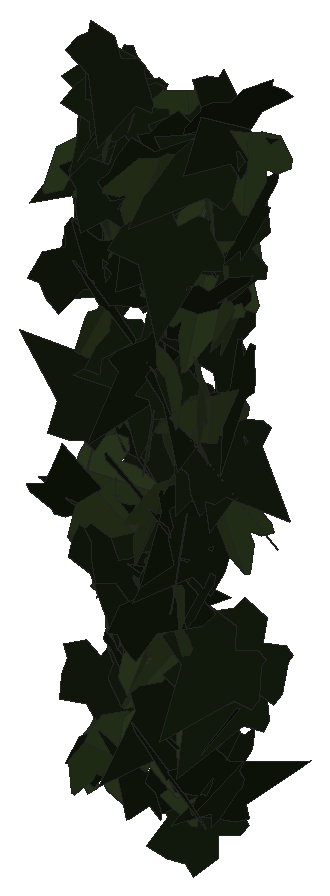
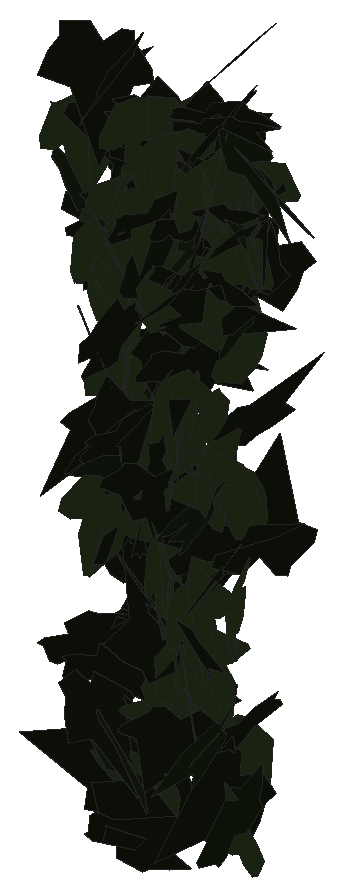
# SketchUp Ruby script. Lengths in inches.
U = 1.inch
M = Sketchup.active_model
def pt(a) = Geom::Point3d.new(a.map { |v| v * U })
def face(e, loops, mat)
  f = e.add_face(loops[0].map { |a| pt(a) })
  loops[1..].each { |l| e.add_face(l.map { |a| pt(a) }).erase! }
  f.material = f.back_material = mat if mat
  f
end
# faces: each face lists its corners as indices into pts; further lists are holes
def faces(e, pts, list, mat = nil) = list.each { |f| face(e, (f[0].is_a?(Array) ? f : [f]).map { |l| l.map { |i| pts[i] } }, mat) }
# xy, xz, yz: faces in a plane at the given z, y or x. An outline is a flat list of corners, or four numbers for a rectangle; further outlines are holes
def ring(l) = l.size == 4 ? [[l[0], l[1]], [l[2], l[1]], [l[2], l[3]], [l[0], l[3]]] : l.each_slice(2).to_a
def flat(e, list, mat, &to3) = list.each { |f| face(e, (f[0].is_a?(Array) ? f : [f]).map { |l| ring(l).map { |u, v| to3.(u, v) } }, mat) }
def xy(e, z, list, mat = nil) = flat(e, list, mat) { |x, y| [x, y, z] }
def xz(e, y, list, mat = nil) = flat(e, list, mat) { |x, z| [x, y, z] }
def yz(e, x, list, mat = nil) = flat(e, list, mat) { |y, z| [x, y, z] }
def lines(e, pts, list) = list.each { |a, b| e.add_line(pt(pts[a]), pt(pts[b])) }
# prism: a flat outline (further loops are holes) pulled along v
def prism(e, loops, v, mat = nil)
  f = face(e, loops, mat); d = Geom::Vector3d.new(v.map { |x| x * U })
  f.pushpull(f.normal.samedirection?(d) ? d.length : -d.length)
end
def box(e, o, s, mat = nil) = prism(e, [[o, [o[0] + s[0], o[1], o[2]], [o[0] + s[0], o[1] + s[1], o[2]], [o[0], o[1] + s[1], o[2]]]], [0, 0, s[2]], mat)
def at(x, y, z, deg = 0) = Geom::Transformation.translation(pt([x, y, z])) * Geom::Transformation.rotation(ORIGIN, Z_AXIS, deg.degrees)
def axes(o, x, y, z) = Geom::Transformation.new([*x, 0, *y, 0, *z, 0, *pt(o).to_a, 1])
def part(name) = M.definitions.add(name)
# library, detail: a bought-in or finely detailed component or shape, given as its bounding box
def library(name, o, s) = part(name).tap { |d| box(d.entities, o, s) }
def detail(e, o, s) = box(e.add_group.entities, o, s)
def put(e, d, t, mat = nil) = e.add_instance(d, t).tap { |i| i.material = mat if mat }
def group(e, t, mat = nil) = e.add_group.tap { |g| g.transformation = t; g.material = mat if mat }.entities
root = M.entities
M.materials.add("efeu1").color = [18, 25, 13]
M.materials.add("efeu2").color = [43, 57, 29]
c1 = part("ivyleaf_9")
p = [[1.54,2.16,1.25],[1.36,2.04,1.19],[-0.21,0.99,0.68],[-0.71,1.11,0.82],[-0.85,0.86,0.67],[-0.8,0.17,0.21],
  [-0.9,-0.01,0.1],[-0.67,-0.16,-0.02],[-0.08,-0.08,-0.05],[-0.03,-0.6,-0.4],[0.65,-0.88,-0.66],[0.83,-0.6,-0.49],
  [1.29,-0.42,-0.43],[1.8125,-0.07,-0.26],[1.21,0.44,0.15]]
faces(c1.entities,p,[[0,1,2,3,4,5,6,7,8,9,10,11,12,13,14]],"efeu1")
c2 = part("ivyleaf_10")
p = [[0,0.5,-0.03],[-0.0625,2.02,-0.43],[-0.19,2.01,-0.46],[-0.54,1.05,-0.29],[-0.52,0.625,-0.18],[-0.83,0.76,-0.28],
  [-1.16,0.64,-0.33],[-1.15,0.33,-0.24],[-0.77,-0.39,0.02],[-0.3,-0.51,0.16],[0.04,-0.48,0.23],[-0.02,2.01,-0.4375],
  [-0.06,2.01,-0.43],[0.04,-0.49,0.23],[0.67,-0.49,0.14],[1.38,0.36,-0.2],[1.375,0.51,-0.24],[0.81,0.65,-0.19],
  [0.62,0.59,-0.15],[0.6,1.09,-0.28],[0.5,1.23,-0.31]]
faces(c2.entities,p,[[0,1,2,3,4,5,6,7,8,9,10],[11,12,0,13,14,15,16,17,18,19,20]],"efeu2")
put(root,c1,axes([33.98,222.86,232.78],[-0.31078,0.3911,-0.0214],[0.01614,-0.01451,-0.49953],[-0.39135,-0.31118,-0.00361]))
put(root,c1,axes([33.44,223.66,223.55],[0.09535,-0.32828,0.36489],[0.19761,-0.31458,-0.33465],[0.44929,0.20803,0.06975]))
put(root,c1,axes([33.7,222.8,227.01],[0.44975,-0.01746,0.21775],[-0.21765,0.00672,0.45009],[-0.01864,-0.49965,-0.00156]))
put(root,c2,axes([33.75,223.1875,231.32],[-0.11704,-0.40418,-0.27008],[0.11553,0.24671,-0.41927],[0.47218,-0.16055,0.03564]))
put(root,c1,axes([33.97,222.84,228.65],[-0.13388,-0.48109,-0.02511],[0.00928,-0.02864,0.49909],[-0.48165,0.13317,0.0166]))
put(root,c2,axes([33.62,223.42,226.43],[0.0575,-0.20142,0.45401],[0.32343,-0.33168,-0.18811],[0.37695,0.31531,0.09215]))
put(root,c2,axes([33.72,222.86,232.22],[-0.17734,-0.45005,-0.12652],[0.25491,0.02034,-0.42966],[0.39188,-0.21689,0.22223]))
put(root,c1,axes([34.16,222.77,232.45],[-0.47089,0.16256,0.04285],[-0.04151,0.01106,-0.49815],[-0.16291,-0.47271,0.00308]))
put(root,c2,axes([34.12,222.57,231.95],[-0.29465,0.19178,0.35553],[-0.32414,0.15037,-0.34975],[-0.24107,-0.43659,0.03572]))
put(root,c1,axes([34.15,223.67,230.54],[-0.34353,-0.21375,0.29377],[-0.25674,-0.14322,-0.40444],[0.25705,-0.42872,-0.01136]))
put(root,c2,axes([34.09,222.84,231.64],[0.32085,-0.20462,-0.32433],[-0.24415,0.2171,-0.3785],[0.29572,0.40125,0.0394]))
put(root,c2,axes([33.57,223.27,223.33],[0.23374,-0.0322,0.44083],[0.43864,-0.04449,-0.23583],[0.05441,0.49697,0.00746]))
put(root,c1,axes([33.8,223.65,231.45],[-0.07618,-0.4723,0.14537],[0.01322,-0.14898,-0.47711],[0.49399,-0.06885,0.03519]))
put(root,c2,axes([33.9,223.49,228.26],[0.07993,-0.28843,0.40052],[0.09701,-0.38864,-0.29924],[0.48394,0.12554,-0.00616]))
put(root,c2,axes([33.62,223.42,228.25],[-0.21577,-0.05871,-0.44721],[0.45021,-0.05834,-0.20955],[-0.02758,-0.4931,0.07804]))
put(root,c2,axes([34.02,223.45,232.32],[-0.14857,-0.46085,0.12468],[-0.00138,-0.13017,-0.48276],[0.47741,-0.14379,0.03741]))
put(root,c1,axes([33.82,222.4,231.03],[0.03859,-0.04451,-0.49652],[-0.03134,0.4968,-0.04697],[0.49752,0.03474,0.03555]))
put(root,c1,axes([33.94,222.95,223.8125],[-0.01726,0.0297,-0.49882],[-0.13859,0.47925,0.03333],[0.4801,0.13942,-0.00831]))
put(root,c1,axes([33.77,223.46,233.25],[0.17542,-0.46663,-0.03851],[-0.00676,0.03859,-0.49846],[0.46817,0.1754,0.00723]))
put(root,c1,axes([33.8,223.1,224.68],[0.09166,-0.48398,-0.08581],[0.00076,0.08743,-0.4923],[0.49153,0.09012,0.01676]))
put(root,c2,axes([34.04,223.23,232.25],[0.12584,-0.4775,0.07846],[0.0075,-0.07913,-0.49364],[0.48385,0.12542,-0.01275]))
put(root,c1,axes([34.07,223.39,233.11],[-0.393,-0.30878,0.01421],[0.06606,-0.10634,-0.48407],[0.30197,-0.37861,0.12438]))
put(root,c2,axes([34.01,222.67,229.6875],[0.09273,-0.39309,0.29475],[-0.0708,0.28613,0.40388],[-0.4862,-0.11664,-0.00259]))
put(root,c1,axes([34.22,222.81,232.11],[0.19644,0.26418,-0.37632],[-0.205,-0.31598,-0.32883],[-0.41156,0.28349,-0.01582]))
put(root,c2,axes([34.27,223.45,225.65],[-0.31309,-0.29968,0.24933],[-0.18334,-0.16902,-0.43338],[0.34403,-0.3628,-0.00405]))
put(root,c1,axes([33.83,223.46,224.76],[0.40375,-0.28622,-0.07115],[-0.04788,0.05542,-0.49461],[0.29102,0.40621,0.01735]))
put(root,c2,axes([34.08,222.98,232.49],[0.16118,-0.38065,-0.28129],[0.0572,0.31064,-0.38759],[0.46984,0.09277,0.14369]))
put(root,c1,axes([34.39,223.34,227.05],[-0.18695,-0.35165,-0.30231],[-0.14302,-0.26634,0.39826],[-0.44113,0.23538,-0.001]))
put(root,c1,axes([34.1,223.72,231.08],[-0.38595,-0.27514,-0.15918],[0.13878,0.07941,-0.47374],[0.28597,-0.40987,0.01507]))
put(root,c1,axes([33.86,223.56,228.01],[0.34409,-0.36153,0.03],[0.02026,-0.02214,-0.4991],[0.3622,0.34468,-0.00059]))
put(root,c1,axes([34.13,223.62,231.85],[-0.30459,-0.39651,-0.00183],[0.04777,-0.03441,-0.49652],[0.39363,-0.30264,0.05884]))
put(root,c2,axes([34.11,223.21,229.01],[0.11557,-0.33878,-0.3491],[0.13179,0.36721,-0.31272],[0.46827,-0.01973,0.17417]))
put(root,c2,axes([34.23,223.47,226.38],[-0.05056,-0.4972,0.01523],[0.00012,-0.01532,-0.49977],[0.49744,-0.05053,0.00167]))
put(root,c2,axes([34.41,223.63,230.9],[-0.29627,-0.26258,0.30541],[-0.22091,-0.21108,-0.39578],[0.33678,-0.36946,0.00906]))
put(root,c1,axes([33.9,222.8,230.42],[0.38987,-0.30614,0.06545],[0.05144,-0.04047,-0.4957],[0.3088,0.39324,-0.00006]))
put(root,c1,axes([34.22,223.18,233.1],[-0.34727,-0.34579,-0.09918],[0.07763,0.06257,-0.48996],[0.35125,-0.35569,0.01023]))
put(root,c2,axes([34.19,222.71,227.35],[-0.25891,-0.33395,-0.26729],[0.17764,0.20028,-0.42229],[0.38912,-0.31363,0.01493]))
put(root,c1,axes([34.12,223.48,231.49],[0.1783,-0.38561,-0.26365],[0.26782,-0.14683,0.39587],[-0.38273,-0.28239,0.15419]))
put(root,c1,axes([34.58,222.73,232.12],[-0.17959,0.42736,0.18739],[-0.16048,0.13197,-0.45478],[-0.43817,-0.22349,0.08977]))
put(root,c2,axes([34.37,222.92,232],[-0.23587,-0.43268,0.0846],[-0.02326,-0.08361,-0.49241],[0.44026,-0.23622,0.01931]))
put(root,c1,axes([34.17,222.99,233.64],[-0.0635,-0.44035,0.22816],[0.05228,-0.23468,-0.4384],[0.49319,-0.03182,0.07584]))
put(root,c1,axes([34.125,222.82,226.64],[0.10476,-0.47783,0.10345],[0.02104,-0.1013,-0.48918],[0.48845,0.10685,-0.00112]))
put(root,c1,axes([34.14,222.95,226.7],[0.2466,-0.41248,-0.138],[-0.07264,0.11735,-0.48058],[0.42885,0.25707,-0.00205]))
put(root,c2,axes([33.97,222.76,227.69],[-0.04468,-0.04275,-0.49616],[0.49663,-0.04072,-0.04122],[-0.03689,-0.4965,0.0461]))
put(root,c1,axes([34.41,223.62,226.06],[-0.45406,-0.05409,-0.20226],[0.20013,0.02978,-0.45723],[0.06151,-0.49617,-0.0054]))
put(root,c2,axes([34.29,222.36,223.95],[-0.13272,-0.29446,-0.38168],[0.19673,0.32833,-0.32171],[0.4401,-0.23557,0.0287]))
put(root,c1,axes([34.11,223.46,231.58],[0.26634,-0.41927,0.05723],[0.04068,-0.04194,-0.49657],[0.4212,0.26917,0.01177]))
put(root,c1,axes([34.08,222.64,230.59],[-0.08991,-0.05781,0.48844],[0.45478,-0.19889,0.06018],[0.18733,0.45509,0.08835]))
put(root,c1,axes([34.17,223.6,230.86],[0.05036,-0.49484,-0.05097],[0.08394,0.05895,-0.48937],[0.49033,0.04073,0.08901]))
put(root,c2,axes([34.62,223.05,225.35],[0.17947,-0.41706,-0.2094],[-0.07988,0.19359,-0.45403],[0.45979,0.19642,0.00286]))
put(root,c1,axes([34.36,223.54,224.72],[-0.13742,-0.35427,-0.32497],[0.14347,0.29236,-0.3794],[0.45884,-0.19752,0.0213]))
put(root,c2,axes([34.57,223.4,229.11],[0.00386,-0.49969,-0.01721],[0.03205,0.01743,-0.49867],[0.49896,0.00274,0.03216]))
put(root,c2,axes([34.76,223.17,228.56],[-0.33587,0.21662,0.30045],[-0.24414,0.17553,-0.39948],[-0.27854,-0.41505,-0.01213]))
put(root,c2,axes([34.5,223.43,232.6875],[0.21454,0.45143,-0.01345],[-0.00632,-0.01189,-0.49982],[-0.45159,0.21463,0.00061]))
put(root,c1,axes([34.46,223.26,231.08],[-0.0479,-0.31294,0.38701],[-0.00586,-0.38841,-0.3148],[0.49767,-0.03469,0.03354]))
put(root,c1,axes([34.5,222.42,232.44],[0.07252,-0.32742,-0.37086],[-0.08288,0.36148,-0.33535],[0.48772,0.11011,-0.00184]))
put(root,c2,axes([34.79,223.29,226],[0.30264,-0.28144,-0.28142],[-0.14495,0.25132,-0.40722],[0.37067,0.32807,0.07053]))
put(root,c1,axes([34.6,223.12,229.58],[-0.1939,-0.44753,-0.11008],[0.04307,0.10131,-0.48773],[0.45885,-0.19863,-0.00074]))
put(root,c2,axes([34.57,223,225.05],[0.06689,0.35995,0.34053],[0.06703,0.33389,-0.36609],[-0.49095,0.09463,-0.00359]))
put(root,c1,axes([34.36,223.07,227.53],[0.10531,-0.33949,0.35165],[0.24873,-0.27244,-0.3375],[0.42076,0.24602,0.1115]))
put(root,c1,axes([34.5,222.89,223.51],[-0.00503,-0.3185,0.3854],[0.11091,-0.37653,-0.30972],[0.48752,0.08238,0.07444]))
put(root,c2,axes([34.61,223.5,226.71],[-0.2528,0.2507,-0.35106],[0.11468,-0.3532,-0.33481],[-0.41586,-0.2498,0.12108]))
put(root,c1,axes([34.45,223.45,225.79],[0.44248,0.23187,-0.02124],[0.01151,0.02376,0.4993],[0.23256,-0.44235,0.01569]))
put(root,c2,axes([34.78,223.35,226.81],[0.06635,-0.4863,-0.09544],[0.01245,0.09789,-0.49017],[0.49542,0.06267,0.0251]))
put(root,c1,axes([34.69,223.6,228.02],[-0.25981,-0.32164,-0.28116],[0.17916,0.2167,-0.41345],[0.38782,-0.31558,0.00264]))
put(root,c2,axes([34.88,223.37,231.7],[-0.42076,-0.2696,-0.01662],[0.01244,0.01139,-0.49972],[0.26982,-0.42094,-0.00288]))
put(root,c2,axes([34.9,222.68,228.79],[0.26857,-0.34606,-0.24107],[-0.07092,0.24467,-0.43024],[0.41574,0.2653,0.08234]))
put(root,c2,axes([34.87,223.55,233],[-0.37519,-0.33049,0.00258],[0.05209,-0.06298,-0.49328],[0.32637,-0.36988,0.08169]))
put(root,c1,axes([34.8125,223.56,231.6875],[-0.2196,-0.4482,0.02988],[-0.00768,-0.02951,-0.49907],[0.44913,-0.21965,0.00607]))
put(root,c1,axes([35.26,222.89,229.62],[-0.39556,0.04584,0.30238],[-0.30379,-0.00196,-0.39712],[-0.03522,-0.49789,0.0294]))
put(root,c1,axes([34.98,223.5,232.43],[-0.42946,-0.25289,-0.04012],[0.03288,0.02322,-0.49838],[0.25393,-0.43071,-0.00331]))
put(root,c1,axes([35,222.82,229.67],[-0.0221,0.15166,-0.47593],[0.06523,-0.47144,-0.15326],[-0.49523,-0.06886,0.00105]))
put(root,c2,axes([34.99,222.64,232.47],[-0.09975,-0.4778,0.10845],[-0.01309,-0.10804,-0.48801],[0.48977,-0.10019,0.00904]))
put(root,c2,axes([34.96,223.13,225.18],[0.04977,0.19306,-0.45853],[-0.13015,-0.43972,-0.19927],[-0.48019,0.13919,0.00649]))
put(root,c2,axes([35.01,222.77,227.69],[0.09068,-0.47929,0.10979],[0.00528,-0.11069,-0.48757],[0.49168,0.08959,-0.01501]))
put(root,c2,axes([35.15,222.68,229.55],[0.37324,-0.14429,-0.29978],[-0.2331,0.20806,-0.39036],[0.2374,0.43115,0.08804]))
put(root,c1,axes([35.28,223.49,228.26],[0.09861,-0.06096,0.48637],[-0.39943,0.27758,0.11577],[-0.28413,-0.41138,0.00604]))
put(root,c1,axes([34.94,223.33,222.97],[0.40169,0.09268,0.28294],[-0.27369,-0.07211,0.41218],[0.11721,-0.48602,-0.0072]))
put(root,c1,axes([35.25,223.34,226.41],[-0.44967,0.2171,-0.0258],[0.023,-0.01171,-0.49933],[-0.21742,-0.45026,0.00055]))
put(root,c1,axes([34.8,222.57,232.11],[0.00317,-0.00977,0.49989],[0.44494,0.22809,0.00164],[-0.22807,0.44484,0.01014]))
put(root,c2,axes([35.11,222.9,228.69],[-0.47845,0.13121,0.06224],[-0.05915,0.01961,-0.4961],[-0.13262,-0.48208,-0.00324]))
put(root,c1,axes([35.375,223.4375,222.61],[-0.44439,-0.19091,-0.12678],[-0.10767,-0.07024,0.48319],[-0.2023,0.45675,0.02132]))
put(root,c1,axes([34.74,223.66,231.02],[0.10907,-0.22372,0.43365],[0.21567,-0.37649,-0.24848],[0.43771,0.24126,0.01437]))
put(root,c1,axes([35.06,222.91,224.51],[0.01449,-0.0779,-0.49368],[0.21633,-0.44425,0.07645],[-0.45055,-0.21581,0.02082]))
put(root,c2,axes([35.27,223.375,228.62],[-0.44942,0.09823,0.19589],[-0.19704,0.01446,-0.45931],[-0.0959,-0.49004,0.02571]))
put(root,c2,axes([34.91,222.85,224.3],[0.3826,0.27334,0.17],[0.13392,0.10496,-0.47016],[-0.29271,0.4053,0.0071]))
put(root,c2,axes([34.97,222.9375,225.7],[-0.42866,0.06849,0.2481],[0.24641,-0.03004,0.43403],[0.07436,0.49437,-0.008]))
put(root,c2,axes([35.26,223.18,230.72],[-0.16768,-0.44953,0.14072],[-0.04973,-0.13164,-0.47979],[0.46841,-0.1749,-0.00056]))
put(root,c1,axes([35.12,222.3,226.42],[0.02515,-0.00424,-0.49935],[-0.14483,0.47843,-0.01136],[0.4779,0.14521,0.02283]))
put(root,c1,axes([34.99,222.48,224.26],[0.44555,-0.20272,-0.10193],[-0.09477,0.03783,-0.48948],[0.20616,0.4555,-0.00472]))
put(root,c2,axes([35.24,223.49,231.85],[0.34407,0.30346,-0.19881],[-0.15541,-0.1243,-0.45869],[-0.32781,0.37744,0.00878]))
put(root,c2,axes([35.07,223.11,227],[0.31917,-0.29864,0.24279],[0.1869,-0.15546,-0.43692],[0.33645,0.36966,0.0124]))
put(root,c1,axes([35.09,223.15,227.28],[0.06739,-0.14142,-0.47482],[0.34038,-0.33498,0.14808],[-0.36,-0.3432,0.05112]))
put(root,c1,axes([35.2,223.67,228.56],[-0.19217,-0.45455,0.08032],[-0.01884,-0.07921,-0.49333],[0.46121,-0.19263,0.01332]))
put(root,c1,axes([34.92,223.21,232.37],[0.13286,-0.03849,0.48048],[0.482,0.0052,-0.13287],[0.00523,0.49849,0.03849]))
put(root,c1,axes([35.61,223.15,223.82],[-0.15078,0.31265,0.35989],[-0.16425,0.32028,-0.34705],[-0.44754,-0.22288,0.00612]))
put(root,c2,axes([35.25,223.48,232.04],[-0.19333,0.44211,-0.131],[0.03139,-0.1291,-0.48202],[-0.46004,-0.1946,0.02216]))
put(root,c2,axes([35.39,223.46,230.83],[0.42202,0.18982,-0.18938],[-0.1806,-0.05982,-0.46239],[-0.1982,0.45868,0.01807]))
put(root,c2,axes([34.9375,223.22,223.42],[0.08412,-0.12107,-0.47777],[0.48208,-0.08068,0.10532],[-0.10259,-0.47837,0.10315]))
put(root,c1,axes([35.52,223.21,232.71],[-0.46012,-0.18162,0.0728],[-0.05764,-0.05198,-0.49394],[0.18699,-0.46294,0.0269]))
put(root,c1,axes([35.11,223.09,228.95],[0.04115,-0.3628,0.34159],[0.09039,-0.33163,-0.36311],[0.49004,0.09164,0.0383]))
put(root,c1,axes([35.35,223.34,227.07],[0.00082,-0.08903,-0.49201],[0.19473,-0.45311,0.08232],[-0.46052,-0.19175,0.03393]))
put(root,c1,axes([35.44,223.83,229.63],[-0.11981,-0.07708,0.47928],[-0.24225,-0.4183,-0.12783],[0.42067,-0.26284,0.06288]))
put(root,c1,axes([35.31,222.74,231.67],[-0.27325,-0.39895,-0.12716],[0.09614,0.08802,-0.48271],[0.40754,-0.28826,0.02861]))
put(root,c1,axes([35.81,223.54,231.24],[-0.33594,-0.05002,0.36694],[-0.3612,-0.06511,-0.33955],[0.08175,-0.49321,0.00761]))
put(root,c2,axes([35.58,223.49,231.07],[-0.19308,-0.44729,0.11246],[-0.03205,-0.10861,-0.48701],[0.4601,-0.19527,0.01327]))
put(root,c2,axes([35.54,223.45,227.37],[-0.49111,-0.07004,-0.06251],[0.06215,0.007,-0.49607],[0.07037,-0.49502,0.00183]))
put(root,c1,axes([35.71,222.87,230.82],[-0.03028,0.40411,-0.29287],[0.00203,-0.29331,-0.40492],[-0.49908,-0.02571,0.01613]))
put(root,c1,axes([35.45,223.68,228.36],[-0.07257,-0.4755,0.13651],[0.01384,-0.13987,-0.47984],[0.49451,-0.06586,0.03346]))
put(root,c2,axes([35.58,222.93,230.74],[0.13401,0.45762,-0.15041],[-0.10185,-0.12568,-0.47311],[-0.47082,0.15744,0.05953]))
put(root,c2,axes([35.68,222.96,229.1],[-0.24045,-0.4383,-0.00881],[-0.0016,0.01093,-0.49988],[0.43838,-0.24036,-0.00666]))
put(root,c1,axes([35.73,223.32,225.39],[-0.33158,-0.35521,0.11783],[-0.08434,-0.08245,-0.48589],[0.36461,-0.3421,-0.00524]))
put(root,c2,axes([35.72,222.6875,229.51],[0.23147,-0.27978,-0.34372],[-0.04901,0.36924,-0.33356],[0.44048,0.18811,0.14351]))
put(root,c1,axes([35.6,223.52,233.0625],[-0.06912,-0.30887,0.38706],[-0.07568,-0.37964,-0.31646],[0.48938,-0.10234,0.00573]))
put(root,c1,axes([35.875,223.34,224.58],[-0.21698,0.41215,-0.1818],[0.08694,-0.15968,-0.46577],[-0.442,-0.23374,-0.00237]))
put(root,c1,axes([35.97,223.125,223.82],[-0.40414,0.29416,-0.01208],[0.00594,-0.01236,-0.49981],[-0.29434,-0.40413,0.0065]))
put(root,c1,axes([35.83,223.21,233.5],[0.11115,0.47821,-0.09464],[-0.02699,-0.09089,-0.49093],[-0.48674,0.11424,0.00561]))
put(root,c1,axes([35.79,223.31,225.03],[-0.36079,-0.34608,0.00768],[-0.00308,-0.00789,-0.49993],[0.34615,-0.36079,0.00357]))
put(root,c2,axes([35.82,223.5625,232.71],[-0.38025,-0.32155,0.04488],[0.01046,-0.08121,-0.49325],[0.3245,-0.37418,0.06849]))
put(root,c1,axes([35.45,223.17,228.17],[0.42177,-0.24931,0.09978],[0.08088,-0.05923,-0.48985],[0.25607,0.42934,-0.00963]))
put(root,c2,axes([35.64,223.52,230.39],[0.023,-0.02995,0.49857],[0.27929,-0.41301,-0.0377],[0.41408,0.28023,-0.00227]))
put(root,c1,axes([35.94,223.64,225.4375],[-0.35527,-0.31527,0.15616],[-0.11706,-0.10336,-0.47499],[0.33178,-0.37406,-0.00037]))
put(root,c1,axes([35.75,223.51,229.5625],[-0.30474,0.00335,-0.39638],[0.39059,-0.08273,-0.30099],[-0.0676,-0.4931,0.04781]))
put(root,c1,axes([35.7,223.14,228.47],[0.10756,-0.25338,-0.41741],[-0.0687,0.41531,-0.26981],[0.48344,0.1154,0.05452]))
put(root,c1,axes([35.54,222.97,223.42],[0.13117,0.00659,0.48244],[0.4715,0.10436,-0.12962],[-0.1024,0.48894,0.02117]))
put(root,c1,axes([36.09,223.52,231.95],[-0.38614,0.29172,-0.12569],[0.09779,-0.07906,-0.48393],[-0.30222,-0.39831,0.004]))
